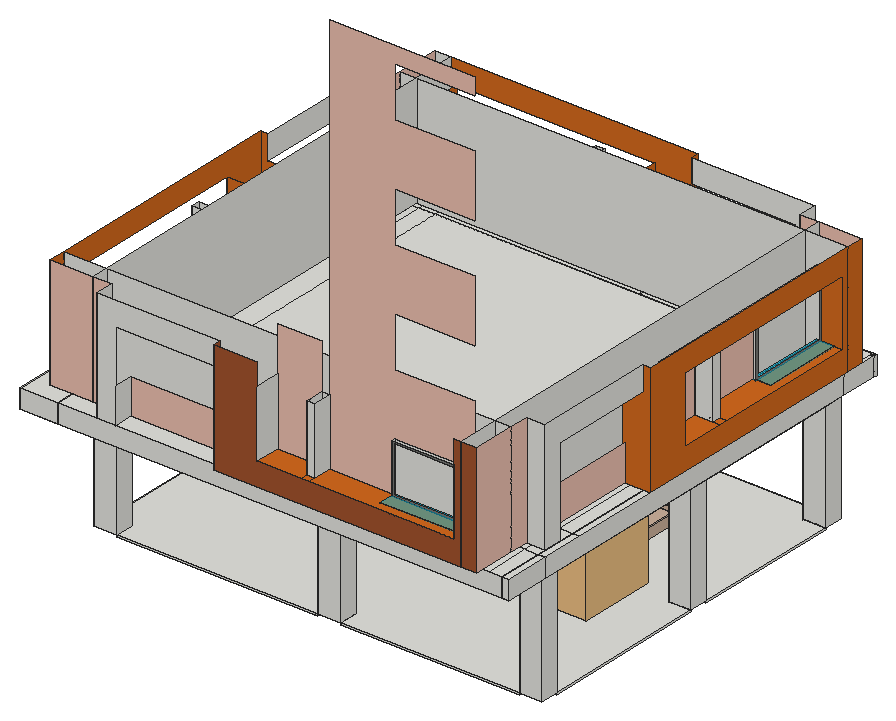
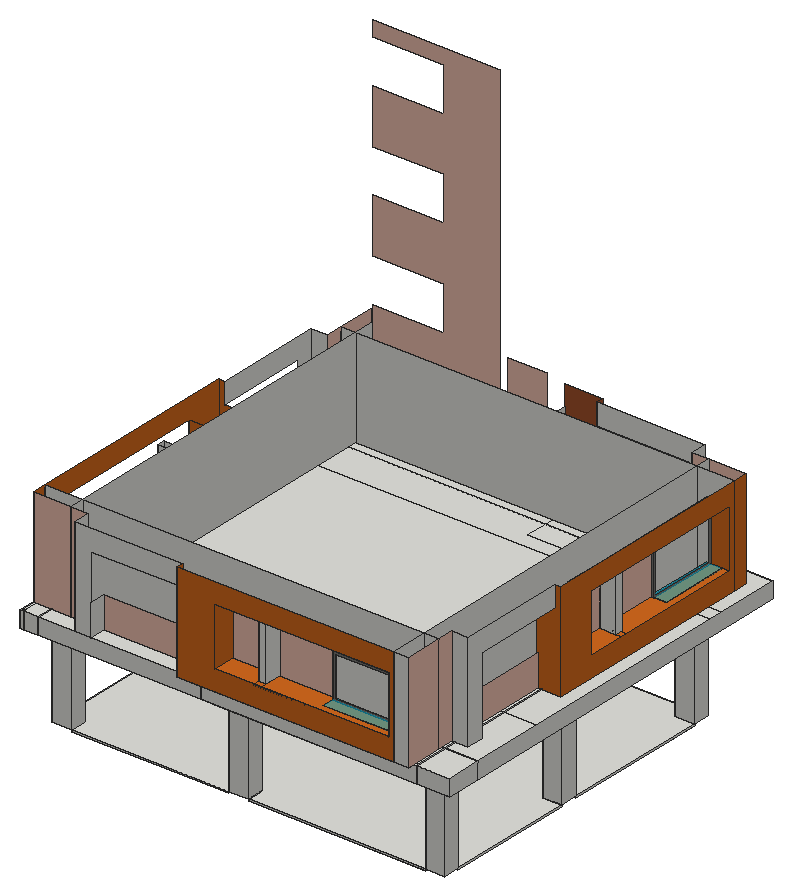
# SketchUp Ruby script. Lengths in inches.
U = 1.inch
M = Sketchup.active_model
def pt(a) = Geom::Point3d.new(a.map { |v| v * U })
def face(e, loops, mat)
  f = e.add_face(loops[0].map { |a| pt(a) })
  loops[1..].each { |l| e.add_face(l.map { |a| pt(a) }).erase! }
  f.material = f.back_material = mat if mat
  f
end
# faces: each face lists its corners as indices into pts; further lists are holes
def faces(e, pts, list, mat = nil) = list.each { |f| face(e, (f[0].is_a?(Array) ? f : [f]).map { |l| l.map { |i| pts[i] } }, mat) }
# xy, xz, yz: faces in a plane at the given z, y or x. An outline is a flat list of corners, or four numbers for a rectangle; further outlines are holes
def ring(l) = l.size == 4 ? [[l[0], l[1]], [l[2], l[1]], [l[2], l[3]], [l[0], l[3]]] : l.each_slice(2).to_a
def flat(e, list, mat, &to3) = list.each { |f| face(e, (f[0].is_a?(Array) ? f : [f]).map { |l| ring(l).map { |u, v| to3.(u, v) } }, mat) }
def xy(e, z, list, mat = nil) = flat(e, list, mat) { |x, y| [x, y, z] }
def xz(e, y, list, mat = nil) = flat(e, list, mat) { |x, z| [x, y, z] }
def yz(e, x, list, mat = nil) = flat(e, list, mat) { |y, z| [x, y, z] }
def lines(e, pts, list) = list.each { |a, b| e.add_line(pt(pts[a]), pt(pts[b])) }
# prism: a flat outline (further loops are holes) pulled along v
def prism(e, loops, v, mat = nil)
  f = face(e, loops, mat); d = Geom::Vector3d.new(v.map { |x| x * U })
  f.pushpull(f.normal.samedirection?(d) ? d.length : -d.length)
end
def box(e, o, s, mat = nil) = prism(e, [[o, [o[0] + s[0], o[1], o[2]], [o[0] + s[0], o[1] + s[1], o[2]], [o[0], o[1] + s[1], o[2]]]], [0, 0, s[2]], mat)
def at(x, y, z, deg = 0) = Geom::Transformation.translation(pt([x, y, z])) * Geom::Transformation.rotation(ORIGIN, Z_AXIS, deg.degrees)
def axes(o, x, y, z) = Geom::Transformation.new([*x, 0, *y, 0, *z, 0, *pt(o).to_a, 1])
def part(name) = M.definitions.add(name)
# library, detail: a bought-in or finely detailed component or shape, given as its bounding box
def library(name, o, s) = part(name).tap { |d| box(d.entities, o, s) }
def detail(e, o, s) = box(e.add_group.entities, o, s)
def put(e, d, t, mat = nil) = e.add_instance(d, t).tap { |i| i.material = mat if mat }
def group(e, t, mat = nil) = e.add_group.tap { |g| g.transformation = t; g.material = mat if mat }.entities
root = M.entities
M.materials.add("Matière par défaut71").color = [191, 191, 191]
M.materials.add("Porta Elevador").color = [142, 142, 142]
M.materials.add("[0041_Chocolate]").color = [210, 105, 30]
M.materials.add("[0042_Sienna]").color = [160, 82, 45]
M.materials.add("[0119_RosyBrown]").color = [234, 190, 174]
M.materials.add("[Color C07]").color = [216, 115, 55]
M.materials.add("[Metal Seamed]").color = [118, 119, 115]
M.materials.add("[Translucent Glass Tinted]").color = [8, 201, 241]
M.materials["[Translucent Glass Tinted]"].alpha = 0.48
M.materials.add("wood").color = [204, 177, 156]
c1 = part("Grouper\#4")
p = [[20.46,2457.84,0.01],[20.52,2457.51,0.05],[20.34,2457.64,0.03],[20.5625,2457.76,0],[20.5625,2492.17,0],[20.35,2492.15,0],
  [20.49,2492.39,0.01],[20.5625,2456.57,0.78],[20.375,2456.28,0.4375],[20.5,2456.62,0.48],[20.5625,2457.16,0.8],[20.5625,2456.91,0.71],
  [20.51,2457.05,0.41],[20.5625,2457.26,0.74],[20.55,2457.2,0.52],[20.5625,2456.66,295.05],[20.5625,2456.98,295.05],[20.53,2457.05,295.67],
  [20.5625,2457.18,295.05],[20.56,2457.1875,295.52],[20.5625,2457.37,295.24],[20.5625,2457.42,295.41],[20.5625,2457.26,295.54],[0,0.81,1592.54],
  [0,0.54,1592.43],[0.07,0.51,1592.89],[0.91,0,1593.5],[0.91,0.18,1593.65],[0.55,0.21,1593.59],[19.9375,0.21,1593.59],
  [19.58,0.18,1593.65],[19.58,0,1593.5]]
faces(c1.entities,p,[[0,1,2],[1,0,3],[4,5,6],[7,8,9],[10,11,12],[13,10,14],[15,16,17],[17,16,18],
  [19,18,20],[20,21,19],[21,22,19],[23,24,25],[26,27,28],[29,30,31]],"Matière par défaut71")
c2 = library("Grouper\#5",[0,0,0],[1856.49,2332.09,3252.59])
c3 = library("Grouper\#1",[0,0,0],[1815.27,2305.3,3203.6])
c4 = part("Grouper\#2")
xy(c4.entities,233.688,[[0,0,849.2,24.21]],"wood")
xy(c4.entities,371.93,[[0,276.347,849.2,298.499]],"wood")
xy(c4.entities,510.172,[[0,552.907,849.2,572.717]],"wood")
xy(c4.entities,904.655,[[0,1456.879,849.2,1733.117]],"wood")
xy(c4.entities,967.358,[[0,1372.402,849.2,1669.765]],"wood")
xy(c4.entities,1063.14,[[0,1648.398,849.2,1668.778]],"wood")
xy(c4.entities,1178.473,[[0,2005.458,849.2,2218.526]],"wood")
xy(c4.entities,1201.382,[[0,1924.882,849.2,1944.274]],"wood")
xy(c4.entities,1233.606,[[32.467,2230.165,2.355,2230.167,2.449,3564.974,32.561,3564.971]],"wood")
xy(c4.entities,1237.805,[[32.637,2219.029,1776.279,3565.134]],"wood")
xy(c4.entities,1241.176,[[0,1924.882,849.2,2218.526]],"wood")
xy(c4.entities,1345.203,[[32.637,2194.999,850.35,2219.029]],"wood")
xy(c4.entities,1383.22,[[931.041,2216.768,1777.375,2279.471]],"wood")
xy(c4.entities,1384.228,[[32.637,2194.999,850.35,2194.999,850.35,2219.029,1776.279,2219.029,1776.279,3565.134,32.637,3565.134]],"wood")
xy(c4.entities,1530.794,[[32.467,2230.165,32.561,3564.971,2.449,3564.974,2.355,2230.167]],"wood")
xy(c4.entities,1531.457,[[1777.031,2392.139,1797.634,2392.139,1797.653,3565.961,1777.05,3565.961]],"wood")
xy(c4.entities,1647.782,[[931.041,2279.471,931.041,2303.681,1777.375,2303.68,1777.375,2279.471]],"wood")
xy(c4.entities,1894.059,[[931.041,2005.181,1777.375,2027.333]],"wood")
xy(c4.entities,2148.052,[[931.041,1730.964,1777.375,1750.773]],"wood")
xz(c4.entities,0,[[0,233.688,849.2,281.086]],"wood")
xz(c4.entities,3.19,[[3.342,0,32.441,342.3125]],"wood")
xz(c4.entities,24.21,[[0,74.417,849.2,233.688]],"wood")
xz(c4.entities,276.347,[[0,371.93,849.2,418.34]],"wood")
xz(c4.entities,298.499,[[0,280.866,849.2,371.93]],"wood")
xz(c4.entities,552.907,[[0,510.172,849.2,555.595]],"wood")
xz(c4.entities,829.021,[[0,648.46,849.2,692.348]],"wood")
xz(c4.entities,847.078,[[0,555.156,849.2,648.368]],"wood")
xz(c4.entities,1105.635,[[0,786.501,849.2,829.116]],"wood")
xz(c4.entities,1109.051,[[1776.98,2508.497,1797.585,2825.325]],"wood")
xz(c4.entities,1121.368,[[0,692.3,849.2,786.415]],"wood")
xz(c4.entities,1372.402,[[0,925.195,849.2,967.358]],"wood")
xz(c4.entities,1395.657,[[0,829.445,849.2,925.102]],"wood")
xz(c4.entities,1456.602,[[931.041,2193.035,1777.375,2392.625]],"wood")
xz(c4.entities,1474.659,[[931.041,2392.718,1777.375,2447.939]],"wood")
xz(c4.entities,1648.398,[[0,1063.14,849.2,1105.6]],"wood")
xz(c4.entities,1750.773,[[931.041,2148.052,1777.375,2193.474]],"wood")
xz(c4.entities,1924.882,[[0,1201.382,849.2,1241.176]],"wood")
xz(c4.entities,1944.274,[[0,1106.587,849.2,1201.382]],"wood")
xz(c4.entities,2005.181,[[931.041,1694.96,1777.375,1894.059]],"wood")
xz(c4.entities,2027.333,[[931.041,1894.059,1777.375,1940.469]],"wood")
xz(c4.entities,2194.999,[[32.637,1345.203,850.35,1384.228]],"wood")
xz(c4.entities,2218.526,[[0,1178.473,849.2,1241.176]],"wood")
xz(c4.entities,2219.029,[[32.637,1237.805,1776.279,1237.805,1776.279,1384.228,850.35,1384.228,850.35,1345.203,32.637,1345.203]],"wood")
xz(c4.entities,2279.471,[[931.041,1383.22,1777.375,1647.782]],"wood")
xz(c4.entities,2392.139,[[1777.031,1238.179,1797.634,1531.457]],"wood")
xz(c4.entities,3565.134,[[32.637,1237.805,1776.279,1384.228]],"wood")
xz(c4.entities,3565.961,[[1777.05,1233.021,1797.653,1531.457]],"wood")
yz(c4.entities,32.637,[[2219.029,1237.805,2219.029,1345.203,2194.999,1345.203,2194.999,1384.228,3565.134,1384.228,3565.134,1237.805]],"wood")
yz(c4.entities,850.35,[[2194.999,1345.203,2219.029,1384.228]],"wood")
yz(c4.entities,1776.279,[[2219.029,1237.805,3565.134,1384.228]],"wood")
p = [[2.355,2230.167,1233.606],[3.342,3.19,0],[3.342,3.19,342.3125],[2.355,2230.167,1530.794],[32.467,2230.165,1233.606],[32.441,3.19,0],
  [32.467,2230.165,1530.794],[32.441,3.19,342.3125],[2.991,3.509,44.607],[2.671,3.825,44.73],[2.965,3.792,44.539],[3.342,3.787,44.459],
  [3.342,3.484,44.57],[32.444,3.787,44.459],[32.444,3.484,44.57],[32.795,3.509,44.607],[32.822,3.792,44.539],[33.115,3.825,44.73],
  [2.964,4.112,44.586],[2.965,3.34,44.845],[2.671,3.505,44.947],[3.342,3.268,44.811],[32.444,3.268,44.811],[32.822,3.34,44.845],
  [33.115,3.505,44.947],[2.644,4.128,44.822],[2.502,3.799,45.036],[33.284,3.799,45.036],[2.429,4.15,45.176],[0,86.912,75.057],
  [849.2,86.912,75.057],[849.2,24.21,74.417],[0,24.21,74.417],[849.2,85.431,218.337],[0,85.431,218.337],[0,361.202,218.117],
  [849.2,361.202,218.117],[0,359.721,355.568],[849.2,359.721,355.568],[0,298.499,280.866],[0,0,281.086],[849.2,0,281.086],
  [849.2,298.499,280.866],[0,635.541,355.239],[849.2,635.541,355.239],[0,634.01,492.798],[849.2,634.01,492.798],[0,572.789,418.011],
  [0,276.347,418.34],[849.2,276.347,418.34],[849.2,572.789,418.011],[0,572.717,510.172],[849.2,572.717,510.172],[0,909.781,492.359],
  [849.2,909.781,492.359],[849.2,908.3,629.635],[0,908.3,629.635],[0,847.078,555.156],[0,552.907,555.595],[849.2,552.907,555.595],
  [849.2,847.078,555.156],[0,1184.07,629.588],[849.2,1184.07,629.588],[0,1182.589,766.485],[849.2,1182.589,766.485],[0,847.078,648.368],
  [849.2,847.078,648.368],[849.2,829.021,648.46],[0,829.021,648.46],[0,1121.368,692.3],[0,829.021,692.348],[849.2,829.021,692.348],
  [849.2,1121.368,692.3],[849.2,1458.36,766.814],[0,1458.36,766.814],[0,1456.879,904.655],[849.2,1456.879,904.655],[849.2,1121.368,786.415],
  [849.2,1105.635,786.501],[0,1105.635,786.501],[0,1121.368,786.415],[849.2,1105.635,829.116],[849.2,1395.657,829.445],[0,1395.657,829.445],
  [0,1105.635,829.116],[0,1733.117,904.655],[0,1730.575,1043.106],[849.2,1730.575,1043.106],[849.2,1733.117,904.655],[0,1372.402,925.195],
  [0,1395.657,925.102],[849.2,1395.657,925.102],[849.2,1372.402,925.195],[0,1668.778,1063.14],[0,1669.765,967.358],[849.2,1669.765,967.358],
  [849.2,1668.778,1063.14],[0,2006.977,1044.094],[849.2,2006.977,1044.094],[0,2005.458,1178.473],[849.2,2005.458,1178.473],[0,1944.274,1106.587],
  [0,1648.398,1105.6],[849.2,1648.398,1105.6],[849.2,1944.274,1106.587],[1797.653,3565.961,1233.021],[1797.634,2392.139,1238.179],[1777.031,2392.139,1238.179],
  [1777.05,3565.961,1233.021],[1777.05,3565.961,1531.457],[1777.031,2392.139,1531.457],[1797.653,3565.961,1531.457],[1797.634,2392.139,1531.457],[2.449,3564.974,1233.606],
  [1797.652,3565.961,1531.465],[2.449,3564.974,1530.794],[2.43,3600.129,1233.606],[1797.634,3601.116,1233.021],[1797.634,3601.105,1233.021],[1797.634,3601.092,1233.021],
  [1797.634,3601.061,1233.021],[1797.634,3601.116,1529.03],[1797.633,3601.116,1531.465],[2.429,3600.129,1530.794],[32.561,3564.971,1233.606],[32.561,3564.971,1530.794],
  [1776.98,1109.051,2508.497],[1776.98,1109.051,2825.325],[1777.03,2392.14,1531.457],[1777.03,2392.14,1238.179],[1797.585,1109.051,2508.497],[1797.585,1109.051,2825.325],
  [1777.375,2216.768,1383.22],[1777.375,2218.25,1632.431],[931.041,2218.25,1632.431],[931.041,2216.768,1383.22],[1777.375,1942.479,1632.212],[931.041,1942.479,1632.212],
  [1777.375,1943.96,1877.696],[931.041,1943.96,1877.696],[1777.375,2303.68,1695.18],[1777.375,2303.68,1647.782],[931.041,2303.681,1647.782],[931.041,2303.681,1695.18],
  [931.041,2005.181,1694.96],[1777.375,2005.181,1694.96],[1777.375,1668.14,1877.367],[931.041,1668.14,1877.367],[1777.375,1669.67,2130.678],[931.041,1669.67,2130.678],
  [1777.375,1730.892,1940.14],[1777.375,2027.333,1940.469],[931.041,2027.333,1940.469],[931.041,1730.892,1940.14],[1777.375,1730.964,2148.052],[931.041,1730.964,2148.052],
  [1777.375,1393.9,2130.239],[931.041,1393.9,2130.239],[1777.375,1395.381,2373.893],[931.041,1395.381,2373.893],[1777.375,1750.773,2193.474],[931.041,1750.773,2193.474],
  [931.041,1456.602,2193.035],[1777.375,1456.602,2193.035],[1777.375,1105.757,2373.845],[1777.375,1107.238,2450.148],[931.041,1107.238,2450.148],[931.041,1105.757,2373.845],
  [931.041,1456.602,2392.625],[931.041,1474.659,2392.718],[1777.375,1474.659,2392.718],[1777.375,1456.602,2392.625],[931.041,1474.659,2447.939],[1777.375,1474.659,2447.939]]
faces(c4.entities,p,[[0,1,2,3],[4,5,1,0],[5,4,6,7],[8,9,10],[11,12,8],[8,10,11],[12,11,13,14],[15,14,13],
  [13,16,15],[15,16,17],[18,10,9],[8,19,20],[8,12,21],[21,19,8],[21,12,14,22],[22,14,15],
  [15,23,22],[15,24,23],[20,9,8],[17,24,15],[9,25,18],[20,26,9],[17,27,24],[9,26,28],
  [28,25,9],[29,30,31,32],[33,30,29,34],[34,35,36,33],[35,37,38,36],[39,40,41,42],[2,7,6,3],[37,43,44,38],
  [43,45,46,44],[47,48,49,50],[51,47,50,52],[53,54,46,45],[55,54,53,56],[57,58,59,60],[56,61,62,55],[61,63,64,62],
  [65,66,67,68],[69,70,71,72],[73,64,63,74],[74,75,76,73],[77,78,79,80],[81,82,83,84],[85,86,87,88],[89,90,91,92],
  [93,94,95,96],[86,97,98,87],[97,99,100,98],[101,102,103,104],[105,106,107,108],[109,108,107,110],[111,112,106,105],[113,105,111,114,115],
  [116,117,118,119,120,105,113],[121,122,114,111,105,120,119,118,117],[117,116,123,122,121],[4,6,3,0],[6,3,0,4],[0,3,115,113],[6,4,124,125],[123,116,113,115],
  [125,124,113,115],[126,127,128,129],[106,130,126,129,107],[131,130,106,112],[106,112,110,128,129,107],[132,133,134,135],[122,123,115,114],[131,112,110,128,127],
  [133,136,137,134],[136,138,139,137],[140,141,142,143],[143,144,145,140],[138,146,147,139],[146,148,149,147],[150,151,152,153],[154,150,153,155],
  [148,156,157,149],[156,158,159,157],[160,161,162,163],[164,165,166,167],[158,164,167,159],[168,169,170,171],[172,166,165,173]],"wood")
c5 = part("Models (R_2) escalier quart tournant")
p = [[937.98,3563.27,1190.31],[937.97,3563.26,1190.42],[937.98,3563.37,1486.12],[937.98,3563.27,1486.34],[937.98,3598.92,1486.34],[937.98,3598.82,1486.12],
  [937.98,3563.49,1486.24],[937.98,3598.7,1486.24],[937.98,3563.37,1190.53],[937.98,3563.49,1190.41],[937.97,3563.4375,1486.34],[937.98,3563.47,1190.5],
  [937.98,3598.72,1486.14],[937.98,3598.92,1190.31],[937.98,3598.89,1190.33],[937.98,3598.82,1190.53],[937.98,3598.91,1190.33],[937.98,3598.86,1190.33],
  [937.98,3563.47,1486.14],[937.96,3598.8,1190.32],[78.3125,3589.58,1487.99],[78.33,3589.59,1488.11],[937.98,3598.72,1190.5],[937.98,3598.7,1190.41]]
lines(c5.entities,p,[[0,1],[2,3],[4,5],[3,6],[7,4],[0,8],[9,0],[3,10],[0,11],[4,12],[13,14],[15,16],
  [13,17],[3,18],[19,13],[20,21],[14,22],[17,23],[16,13]])
put(c5.entities,c1,at(917.42,1106.01,1190.31))
put(c5.entities,c2,at(-885.67,-8.88,-0.86))
put(c5.entities,c3,at(-867.875,-0.55,-0.86))
put(c5.entities,c4,at(-859.65,-2.2,-42.6875))
c6 = library("Porta Elevador",[0,0,0],[43.31,5.25,90.55])
c7 = part("Altan")
box(c7.entities,[0,0,0],[118.11,59.06,3.9375])
xy(root,-5.6875,[[[192,183.875,192,243.875,120,243.875,120,783.875,188.8125,783.875,188.8125,851.07,120,851.07,120,1323.875,192,1323.875,192,1383.875,840,1383.875,840,1323.875,912,1323.875,912,1383.875,1488,1383.875,1488,1323.875,1560,1323.875,1560,843.875,1488,843.875,1488,783.875,1560,783.875,1560,243.875,1488,243.875,1488,183.875,912,183.875,912,243.875,840,243.875,840,183.875],[912,577.47,1152,577.47,1152,817.47,840,817.47,840,757.47,912,757.47]]])
xy(root,0,[[[192,183.875,840,183.875,840,243.875,912,243.875,912,183.875,1488,183.875,1488,243.875,1560,243.875,1560,783.875,1488,783.875,1488,843.875,1560,843.875,1560,1323.875,1488,1323.875,1488,1383.875,912,1383.875,912,1323.875,840,1323.875,840,1383.875,192,1383.875,192,1323.875,120,1323.875,120,851.07,188.8125,851.07,188.8125,783.875,120,783.875,120,243.875,192,243.875],[912,577.47,912,757.47,840,757.47,840,817.47,1152,817.47,1152,577.47]],[840,183.875,912,243.875],[1488,183.875,1560,243.875],[912,577.47,1152,817.47],[840,757.47,912,817.47],
  [120,783.875,188.8125,851.07],[1488,783.875,1560,843.875],[840,1323.875,912,1383.875]])
xy(root,360,[[0,36.8125,120,243.875],[120,36.8125,192,183.875],[192,36.8125,840,183.875],[840,36.8125,912,183.875],[912,36.8125,1488,183.875],
  [1488,36.8125,1548,183.875],[1548,36.8125,1572,183.875],[120,183.875,192,243.875],[840,183.875,912,243.875],[1488,183.875,1548,243.875],
  [1548,183.875,1560,243.875],[1560,183.875,1572,243.875],[0,243.875,120,783.875],[1548,243.875,1572,783.875],[840,757.47,912,817.47],
  [0,783.875,120,851.07],[120,783.875,188.8125,851.07],[1488,783.875,1548,843.875],[1548,783.875,1560,843.875],[1560,783.875,1572,843.875],
  [1548,843.875,1572,1323.875],[0,851.07,120,1323.875],[0,1323.875,120,1383.875],[120,1323.875,192,1383.875],[840,1323.875,912,1383.875],
  [1488,1323.875,1548,1383.875],[1548,1323.875,1560,1383.875],[1560,1323.875,1572,1383.875],[0,1383.875,120,1512.8125],[120,1383.875,192,1503.875],
  [192,1383.875,840,1503.875],[840,1383.875,912,1503.875],[912,1383.875,1506.3125,1512.8125],[1506.3125,1383.875,1560,1512.8125],[1560,1383.875,1572,1503.875],
  [120,1503.875,192,1512.8125],[192,1503.875,840,1512.8125],[840,1503.875,912,1512.8125],[1560,1503.875,1572,1512.8125]])
xy(root,360,[[[192,183.875,840,183.875,840,243.875,912,243.875,912,183.875,1488,183.875,1488,243.875,1548,243.875,1548,783.875,1488,783.875,1488,843.875,1548,843.875,1548,1323.875,1488,1323.875,1488,1383.875,912,1383.875,912,1323.875,840,1323.875,840,1383.875,192,1383.875,192,1323.875,120,1323.875,120,851.07,188.8125,851.07,188.8125,783.875,120,783.875,120,243.875,192,243.875],[912,577.47,1152,817.47]],[912,577.47,1152,817.47]],"[Color C07]")
xy(root,420,[[0,36.8125,120,267.875],[120,36.8125,713.22,183.875],[713.22,36.8125,1506.3125,183.875],[1506.3125,36.8125,1548,183.875],[1548,36.8125,1572,183.875],
  [120,183.875,713.22,183.875,713.22,267.875,378.65,267.875,378.65,207.875,318.65,207.875,318.65,267.875,120,267.875],[713.22,183.875,1506.3125,183.875,1506.3125,321.5625,1548,321.5625,1548,1383.875,1506.3125,1383.875,1506.3125,321.5625,257.6875,321.5625,257.6875,267.875,318.65,267.875,318.65,207.875,378.65,207.875,378.65,267.875,713.22,267.875],[1506.3125,183.875,1548,321.5625],[1548,183.875,1572,321.5625],[0,267.875,120,321.5625],
  [120,267.875,257.6875,321.5625],[0,321.5625,120,1114.66],[120,321.5625,120,1114.66,204,1114.66,204,1383.875,257.6875,1383.875,257.6875,321.5625],[257.6875,321.5625,1506.3125,1383.875],[1548,321.5625,1572,1383.875],
  [1488,606.03,1488,1212.8125,1434.3125,1212.8125,1434.3125,1399.125,1572,1399.125,1572,606.03],[0,1114.66,120,1383.875],[120,1114.66,204,1383.875],[132,1212.8125,132,1278.16,72,1278.16,72,1338.16,132,1338.16,132,1399.125,185.6875,1399.125,185.6875,1212.8125],[0,1383.875,120,1512.8125],
  [120,1383.875,204,1503.875],[204,1383.875,257.6875,1503.875],[257.6875,1383.875,912,1503.875],[912,1383.875,1506.3125,1512.8125],[1506.3125,1383.875,1560,1512.8125],
  [1560,1383.875,1572,1503.875],[132,1399.125,185.6875,1536.8125],[185.6875,1399.125,185.6875,1536.8125,978.78,1536.8125,978.78,1452.8125,1313.35,1452.8125,1313.35,1512.8125,1373.35,1512.8125,1373.35,1452.8125,1434.3125,1452.8125,1434.3125,1399.125],[120,1503.875,204,1512.8125],[204,1503.875,257.6875,1512.8125],
  [257.6875,1503.875,912,1512.8125],[1560,1503.875,1572,1512.8125]])
xy(root,493.11,[[922.01,36.8125,948.52,96.8125],[72,636.29,132,662.8],[1488,886.83,1548,913.33],[671.48,1452.8125,697.99,1512.8125]])
xy(root,493.11,[[778.64,12.8125,922.01,96.8125],[922.01,12.8125,948.52,36.8125],[948.52,12.8125,1414.89,12.8125,1414.89,84.8125,1155.2,84.8125,1155.2,96.8125,948.52,96.8125],[48,169.92,120,169.92,120,429.61,132,429.61,132,636.29,48,636.29],[48,636.29,72,662.8],
  [48,662.8,132,806.17],[1488,743.45,1572,886.83],[1548,886.83,1572,913.33],[1488,913.33,1572,913.33,1572,1379.7,1500,1379.7,1500,1120.01,1488,1120.01],[464.8,1452.8125,671.48,1452.8125,671.48,1536.8125,205.11,1536.8125,205.11,1464.8125,464.8,1464.8125],
  [697.99,1452.8125,841.36,1536.8125],[671.48,1512.8125,697.99,1536.8125]],"[0041_Chocolate]")
xz(root,12.8125,[[641.22,420,1434.3125,420,1434.3125,780,1414.89,780,1414.89,493.11,778.64,493.11,778.64,780,641.22,780],[1434.3125,420,1488,780]],"[0042_Sienna]")
xz(root,36.8125,[[0,360,120,420],[120,360,1548,420],[1548,360,1572,420],[246.65,420,306.65,420,306.65,702.625,641.22,702.625,641.22,780,246.65,780],[922.01,493.11,948.52,706.89]])
xz(root,84.8125,[[[1155.2,493.11,1414.89,653.61],[1161.2,499.11,1408.89,647.61]]],"[Metal Seamed]")
xz(root,96.8125,[[922.01,493.11,948.52,706.89]])
xz(root,96.8125,[[48,420,185.6875,780],[185.6875,420,246.65,780],[306.65,420,641.22,533.76],[778.64,493.11,922.01,853.11],[948.52,493.11,1155.2,493.11,1155.2,653.61,1414.89,653.61,1414.89,853.11,1155.2,853.11,1155.2,1013.61,1414.89,1013.61,1414.89,1213.11,1155.2,1213.11,1155.2,1373.61,1414.89,1373.61,1414.89,1573.11,1155.2,1573.11,1155.2,1733.61,1414.89,1733.61,1414.89,1786.89,948.52,1786.89]],"[0119_RosyBrown]")
xz(root,150.5,[[48,420,1488,780]])
xz(root,169.92,[[48,493.11,48,706.89,132,706.89,132,653.61,120,653.61,120,493.11]],"[0041_Chocolate]")
xz(root,183.875,[[192,-5.6875,840,0],[912,-5.6875,1488,0],[120,0,192,360],[840,0,912,360],[1488,0,1560,360],
  [120,360,1548,420],[1548,360,1572,420]])
xz(root,211.46,[[1488,420,1548,780]])
xz(root,243.875,[[120,-5.6875,192,360],[840,-5.6875,912,0],[1488,-5.6875,1560,0],[840,0,912,360],[1488,0,1560,360]])
xz(root,271.47,[[1488,420,1548,533.76]])
xz(root,429.61,[[120,493.11,132,653.61]],"[Metal Seamed]")
xz(root,577.47,[[912,-5.6875,1152,0]])
xz(root,577.47,[[912,0,1152,360]],"[0042_Sienna]")
xz(root,606.03,[[1488,420,1572,420,1572,780,1548,780,1548,702.625,1482,702.625,1482,533.76,1488,533.76]],"[0041_Chocolate]")
xz(root,636.29,[[72,493.11,132,706.89]])
xz(root,662.8,[[[72,493.11,132,706.89],[83.53,498.02,84.48,498.14,85.37,498.51,86.13,499.1,86.72,499.86,87.09,500.75,87.21,501.7,87.09,502.66,86.72,503.55,86.13,504.3125,85.37,504.9,84.48,505.27,83.53,505.39,82.57,505.27,81.68,504.9,80.92,504.3125,80.33,503.55,79.97,502.66,79.84,501.7,79.97,500.75,80.33,499.86,80.92,499.1,81.68,498.51,82.57,498.14]]])
xz(root,743.45,[[[1488,493.11,1572,706.89],[1536.47,498.02,1537.43,498.14,1538.32,498.51,1539.08,499.1,1539.67,499.86,1540.03,500.75,1540.16,501.7,1540.03,502.66,1539.67,503.55,1539.08,504.3125,1538.32,504.9,1537.43,505.27,1536.47,505.39,1535.52,505.27,1534.63,504.9,1533.87,504.3125,1533.28,503.55,1532.91,502.66,1532.79,501.7,1532.91,500.75,1533.28,499.86,1533.87,499.1,1534.63,498.51,1535.52,498.14]]],"[0041_Chocolate]")
xz(root,757.47,[[840,-5.6875,912,0],[840,0,912,360]])
xz(root,783.875,[[120,-5.6875,188.8125,0],[1488,-5.6875,1560,0],[120,0,188.8125,360],[1488,0,1560,360]])
xz(root,806.17,[[[48,493.11,132,706.89],[83.53,498.02,82.57,498.14,81.68,498.51,80.92,499.1,80.33,499.86,79.97,500.75,79.84,501.7,79.97,502.66,80.33,503.55,80.92,504.3125,81.68,504.9,82.57,505.27,83.53,505.39,84.48,505.27,85.37,504.9,86.13,504.3125,86.72,503.55,87.09,502.66,87.21,501.7,87.09,500.75,86.72,499.86,86.13,499.1,85.37,498.51,84.48,498.14]]],"[0041_Chocolate]")
xz(root,817.47,[[840,-5.6875,912,0],[912,-5.6875,1152,0],[840,0,912,360]])
xz(root,817.47,[[912,0,1152,360]],"[Color C07]")
xz(root,843.875,[[1488,-5.6875,1560,0],[1488,0,1560,360]])
xz(root,851.07,[[120,-5.6875,188.8125,0],[120,0,188.8125,360]])
xz(root,886.83,[[[1488,493.11,1548,706.89],[1536.47,498.02,1535.52,498.14,1534.63,498.51,1533.87,499.1,1533.28,499.86,1532.91,500.75,1532.79,501.7,1532.91,502.66,1533.28,503.55,1533.87,504.3125,1534.63,504.9,1535.52,505.27,1536.47,505.39,1537.43,505.27,1538.32,504.9,1539.08,504.3125,1539.67,503.55,1540.03,502.66,1540.16,501.7,1540.03,500.75,1539.67,499.86,1539.08,499.1,1538.32,498.51,1537.43,498.14]]])
xz(root,913.33,[[1488,493.11,1548,706.89]])
xz(root,943.59,[[48,420,48,780,72,780,72,702.625,138,702.625,138,533.76,132,533.76,132,420]],"[0041_Chocolate]")
xz(root,1120.01,[[1488,493.11,1500,653.61]])
xz(root,1278.16,[[72,420,132,533.76]])
xz(root,1323.875,[[120,-5.6875,192,360],[840,-5.6875,912,0],[1488,-5.6875,1560,0],[840,0,912,360],[1488,0,1560,360]])
xz(root,1338.16,[[72,420,132,780]])
xz(root,1379.7,[[1500,493.11,1572,493.11,1572,706.89,1488,706.89,1488,653.61,1500,653.61]],"[0041_Chocolate]")
xz(root,1383.875,[[192,-5.6875,840,0],[912,-5.6875,1488,0],[120,0,192,360],[840,0,912,360],[1488,0,1560,360],
  [0,360,120,420],[120,360,912,420],[912,360,1506.3125,420],[1506.3125,360,1548,420],[1548,360,1572,420]])
xz(root,1399.125,[[132,420,1572,780]])
xz(root,1452.8125,[[671.48,493.11,697.99,706.89]])
xz(root,1452.8125,[[978.78,420,1313.35,533.76],[1373.35,420,1434.3125,780],[1434.3125,420,1572,780],[464.8,493.11,464.8,653.61,205.11,653.61,205.11,706.89,671.48,706.89,671.48,493.11],[697.99,493.11,841.36,706.89]],"[0119_RosyBrown]")
xz(root,1464.8125,[[[205.11,493.11,464.8,653.61],[211.11,499.11,458.8,647.61]]],"[Metal Seamed]")
xz(root,1503.875,[[120,360,912,420],[1560,360,1572,420]])
xz(root,1512.8125,[[0,360,120,420],[120,360,912,420],[912,360,1506.3125,420],[1506.3125,360,1560,420],[1560,360,1572,420],
  [1313.35,420,1313.35,702.625,978.78,702.625,978.78,780,1373.35,780,1373.35,420],[671.48,493.11,697.99,706.89]])
xz(root,1536.8125,[[132,420,185.6875,780]])
xz(root,1536.8125,[[[185.6875,420,978.78,780],[205.11,493.11,841.36,706.89]]],"[0041_Chocolate]")
yz(root,0,[[36.8125,360,1383.875,420],[1383.875,360,1512.8125,420]])
yz(root,48,[[96.8125,420,150.5,780],[[150.5,420,943.59,780],[169.92,493.11,806.17,706.89]]],"[0041_Chocolate]")
yz(root,72,[[1278.16,420,1278.16,702.625,943.59,702.625,943.59,780,1338.16,780,1338.16,420],[636.29,493.11,662.8,706.89]])
yz(root,120,[[243.875,-5.6875,783.875,0],[851.07,-5.6875,1323.875,0],[183.875,0,243.875,360],[783.875,0,851.07,360],[1323.875,0,1383.875,360],
  [36.8125,360,183.875,420],[183.875,360,1383.875,420],[1383.875,360,1503.875,420],[1503.875,360,1512.8125,420]])
yz(root,120,[[[169.92,493.11,429.61,653.61],[175.92,499.11,423.61,647.61]]],"[Metal Seamed]")
yz(root,132,[[636.29,493.11,662.8,706.89]])
yz(root,132,[[943.59,420,1278.16,533.76],[1338.16,420,1399.125,780],[1399.125,420,1536.8125,780],[429.61,493.11,429.61,653.61,169.92,653.61,169.92,706.89,636.29,706.89,636.29,493.11],[662.8,493.11,806.17,706.89]],"[0119_RosyBrown]")
yz(root,185.6875,[[96.8125,420,1536.8125,780]])
yz(root,188.8125,[[783.875,-5.6875,851.07,0],[783.875,0,851.07,360]])
yz(root,192,[[183.875,-5.6875,243.875,360],[1323.875,-5.6875,1383.875,360]])
yz(root,205.11,[[1464.8125,493.11,1536.8125,493.11,1536.8125,706.89,1452.8125,706.89,1452.8125,653.61,1464.8125,653.61]],"[0041_Chocolate]")
yz(root,246.65,[[36.8125,420,96.8125,780]])
yz(root,306.65,[[36.8125,420,96.8125,533.76]])
yz(root,464.8,[[1452.8125,493.11,1464.8125,653.61]])
yz(root,641.22,[[12.8125,420,12.8125,780,36.8125,780,36.8125,702.625,102.8125,702.625,102.8125,533.76,96.8125,533.76,96.8125,420]],"[0042_Sienna]")
yz(root,671.48,[[1452.8125,493.11,1512.8125,706.89]])
yz(root,697.99,[[[1452.8125,493.11,1512.8125,706.89],[1501.28,498.02,1500.33,498.14,1499.44,498.51,1498.68,499.1,1498.09,499.86,1497.72,500.75,1497.6,501.7,1497.72,502.66,1498.09,503.55,1498.68,504.3125,1499.44,504.9,1500.33,505.27,1501.28,505.39,1502.24,505.27,1503.13,504.9,1503.89,504.3125,1504.48,503.55,1504.85,502.66,1504.97,501.7,1504.85,500.75,1504.48,499.86,1503.89,499.1,1503.13,498.51,1502.24,498.14]]])
yz(root,778.64,[[[12.8125,493.11,96.8125,493.11,96.8125,706.89,51.8,706.89,51.9,706.66,52.03,705.7,51.9,704.75,51.53,703.86,50.95,703.1,50.18,702.51,49.29,702.14,48.34,702.02,47.38,702.14,46.5,702.51,45.73,703.1,45.15,703.86,44.78,704.75,44.65,705.7,44.78,706.66,44.875,706.89,12.8125,706.89],[48.34,498.02,47.38,498.14,46.5,498.51,45.73,499.1,45.15,499.86,44.78,500.75,44.65,501.7,44.78,502.66,45.15,503.55,45.73,504.3125,46.5,504.9,47.38,505.27,48.34,505.39,49.29,505.27,50.18,504.9,50.95,504.3125,51.53,503.55,51.9,502.66,52.03,501.7,51.9,500.75,51.53,499.86,50.95,499.1,50.18,498.51,49.29,498.14]]])
yz(root,840,[[183.875,-5.6875,243.875,0],[757.47,-5.6875,817.47,0],[1323.875,-5.6875,1383.875,0],[183.875,0,243.875,360],[757.47,0,817.47,360],
  [1323.875,0,1383.875,360]])
yz(root,841.36,[[[1452.8125,493.11,1536.8125,706.89],[1501.28,498.02,1502.24,498.14,1503.13,498.51,1503.89,499.1,1504.48,499.86,1504.85,500.75,1504.97,501.7,1504.85,502.66,1504.48,503.55,1503.89,504.3125,1503.13,504.9,1502.24,505.27,1501.28,505.39,1500.33,505.27,1499.44,504.9,1498.68,504.3125,1498.09,503.55,1497.72,502.66,1497.6,501.7,1497.72,500.75,1498.09,499.86,1498.68,499.1,1499.44,498.51,1500.33,498.14]]],"[0041_Chocolate]")
yz(root,912,[[183.875,-5.6875,243.875,0],[577.47,-5.6875,757.47,0],[1323.875,-5.6875,1383.875,0],[183.875,0,243.875,360],[757.47,0,817.47,360],
  [1323.875,0,1383.875,360],[1383.875,360,1503.875,420],[1503.875,360,1512.8125,420]])
yz(root,912,[[577.47,0,757.47,360]],"[Color C07]")
yz(root,922.01,[[[36.8125,493.11,36.8125,706.89,44.875,706.89,44.78,706.66,44.65,705.7,44.78,704.75,45.15,703.86,45.73,703.1,46.5,702.51,47.38,702.14,48.34,702.02,49.29,702.14,50.18,702.51,50.95,703.1,51.53,703.86,51.9,704.75,52.03,705.7,51.9,706.66,51.8,706.89,96.8125,706.89,96.8125,493.11],[48.34,498.02,49.29,498.14,50.18,498.51,50.95,499.1,51.53,499.86,51.9,500.75,52.03,501.7,51.9,502.66,51.53,503.55,50.95,504.3125,50.18,504.9,49.29,505.27,48.34,505.39,47.38,505.27,46.5,504.9,45.73,504.3125,45.15,503.55,44.78,502.66,44.65,501.7,44.78,500.75,45.15,499.86,45.73,499.1,46.5,498.51,47.38,498.14]]])
yz(root,948.52,[[36.8125,493.11,96.8125,706.89]])
yz(root,978.78,[[1452.8125,420,1536.8125,420,1536.8125,780,1512.8125,780,1512.8125,702.625,1446.8125,702.625,1446.8125,533.76,1452.8125,533.76]],"[0041_Chocolate]")
yz(root,1152,[[577.47,-5.6875,817.47,0]])
yz(root,1152,[[577.47,0,817.47,360]],"[Color C07]")
yz(root,1155.2,[[84.8125,493.11,96.8125,653.61]])
yz(root,1313.35,[[1452.8125,420,1512.8125,533.76]])
yz(root,1373.35,[[1452.8125,420,1512.8125,780]])
yz(root,1414.89,[[12.8125,493.11,12.8125,706.89,96.8125,706.89,96.8125,653.61,84.8125,653.61,84.8125,493.11]],"[0041_Chocolate]")
yz(root,1434.3125,[[12.8125,420,1452.8125,780]])
yz(root,1488,[[183.875,-5.6875,243.875,0],[783.875,-5.6875,843.875,0],[1323.875,-5.6875,1383.875,360],[183.875,0,243.875,360],[783.875,0,843.875,360],
  [886.83,493.11,913.33,706.89]])
yz(root,1488,[[12.8125,420,150.5,780],[150.5,420,211.46,780],[271.47,420,606.03,533.76],[743.45,493.11,886.83,706.89],[913.33,493.11,1120.01,493.11,1120.01,653.61,1379.7,653.61,1379.7,706.89,913.33,706.89]],"[0119_RosyBrown]")
yz(root,1500,[[[1120.01,493.11,1379.7,653.61],[1126.01,499.11,1373.7,647.61]]],"[Metal Seamed]")
yz(root,1506.3125,[[1383.875,360,1512.8125,420]])
yz(root,1548,[[36.8125,360,183.875,420],[183.875,360,1383.875,420],[211.46,420,271.47,420,271.47,702.625,606.03,702.625,606.03,780,211.46,780],[886.83,493.11,913.33,706.89]])
yz(root,1560,[[243.875,-5.6875,783.875,0],[843.875,-5.6875,1323.875,0],[183.875,0,243.875,360],[783.875,0,843.875,360],[1323.875,0,1383.875,360],
  [1503.875,360,1512.8125,420]])
yz(root,1572,[[36.8125,360,183.875,420],[183.875,360,1383.875,420],[1383.875,360,1503.875,420],[1503.875,360,1512.8125,420]])
yz(root,1572,[[[606.03,420,1399.125,780],[743.45,493.11,1379.7,706.89]],[1399.125,420,1452.8125,780]],"[0041_Chocolate]")
put(root,c5,axes([1264.01,578.42,-7.2],[0.12647,0,0],[0,0.10604,0],[0,0,0.1068]))
put(root,c6,axes([927.78,817.47,0],[2.2213,0,0],[0,2.2213,0],[0,0,2.2213]))
put(root,c7,axes([205.11,1451.94,489.17],[2.19843,0,0],[0,1,0],[0,0,1.5]),"[Translucent Glass Tinted]")
put(root,c7,axes([1487.13,1379.7,489.17],[0,-2.19843,0],[1,0,0],[0,0,1.5]),"[Translucent Glass Tinted]")
put(root,c7,axes([1414.89,97.68,489.17],[-2.19843,0,0],[0,-1,0],[0,0,1.5]),"[Translucent Glass Tinted]")
put(root,c7,axes([132.87,169.92,489.17],[0,2.19843,0],[-1,0,0],[0,0,1.5]),"[Translucent Glass Tinted]")
